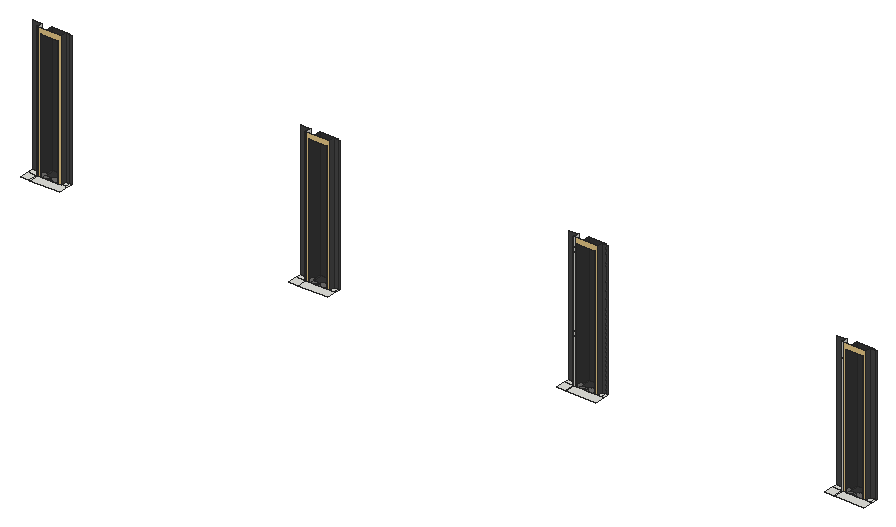
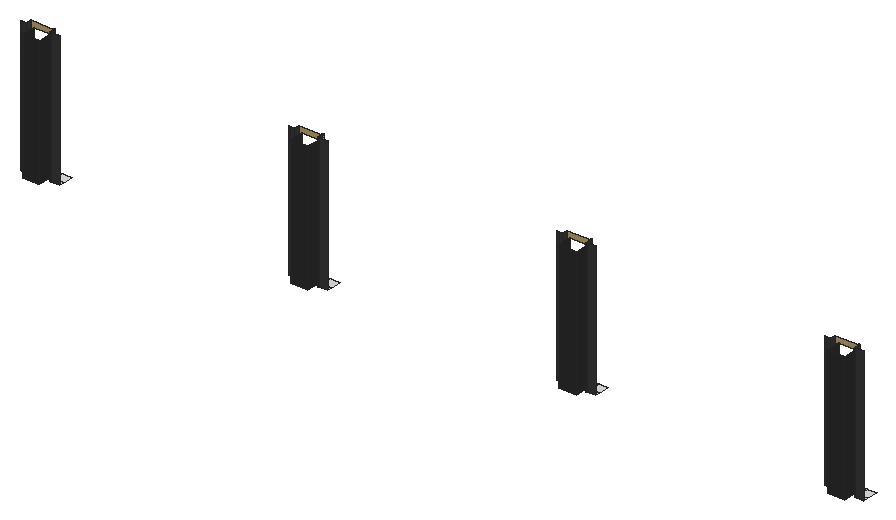
# SketchUp Ruby script. Lengths in inches.
U = 1.inch
M = Sketchup.active_model
def pt(a) = Geom::Point3d.new(a.map { |v| v * U })
def face(e, loops, mat)
  f = e.add_face(loops[0].map { |a| pt(a) })
  loops[1..].each { |l| e.add_face(l.map { |a| pt(a) }).erase! }
  f.material = f.back_material = mat if mat
  f
end
# faces: each face lists its corners as indices into pts; further lists are holes
def faces(e, pts, list, mat = nil) = list.each { |f| face(e, (f[0].is_a?(Array) ? f : [f]).map { |l| l.map { |i| pts[i] } }, mat) }
# xy, xz, yz: faces in a plane at the given z, y or x. An outline is a flat list of corners, or four numbers for a rectangle; further outlines are holes
def ring(l) = l.size == 4 ? [[l[0], l[1]], [l[2], l[1]], [l[2], l[3]], [l[0], l[3]]] : l.each_slice(2).to_a
def flat(e, list, mat, &to3) = list.each { |f| face(e, (f[0].is_a?(Array) ? f : [f]).map { |l| ring(l).map { |u, v| to3.(u, v) } }, mat) }
def xy(e, z, list, mat = nil) = flat(e, list, mat) { |x, y| [x, y, z] }
def xz(e, y, list, mat = nil) = flat(e, list, mat) { |x, z| [x, y, z] }
def yz(e, x, list, mat = nil) = flat(e, list, mat) { |y, z| [x, y, z] }
def lines(e, pts, list) = list.each { |a, b| e.add_line(pt(pts[a]), pt(pts[b])) }
# prism: a flat outline (further loops are holes) pulled along v
def prism(e, loops, v, mat = nil)
  f = face(e, loops, mat); d = Geom::Vector3d.new(v.map { |x| x * U })
  f.pushpull(f.normal.samedirection?(d) ? d.length : -d.length)
end
def box(e, o, s, mat = nil) = prism(e, [[o, [o[0] + s[0], o[1], o[2]], [o[0] + s[0], o[1] + s[1], o[2]], [o[0], o[1] + s[1], o[2]]]], [0, 0, s[2]], mat)
def at(x, y, z, deg = 0) = Geom::Transformation.translation(pt([x, y, z])) * Geom::Transformation.rotation(ORIGIN, Z_AXIS, deg.degrees)
def axes(o, x, y, z) = Geom::Transformation.new([*x, 0, *y, 0, *z, 0, *pt(o).to_a, 1])
def part(name) = M.definitions.add(name)
# library, detail: a bought-in or finely detailed component or shape, given as its bounding box
def library(name, o, s) = part(name).tap { |d| box(d.entities, o, s) }
def detail(e, o, s) = box(e.add_group.entities, o, s)
def put(e, d, t, mat = nil) = e.add_instance(d, t).tap { |i| i.material = mat if mat }
def group(e, t, mat = nil) = e.add_group.tap { |g| g.transformation = t; g.material = mat if mat }.entities
root = M.entities
M.materials.add("[0043_SaddleBrown]4").color = [124, 123, 122]
M.materials.add("[Granite Dark Gray]").color = [69, 68, 68]
M.materials.add("[Slate Light Tile]").color = [54, 54, 54]
M.materials.add("[Stone Brushed Khaki]").color = [226, 197, 133]
xy(root,161.375,[[310,542.125,351.59,589.17],[351.59,542.125,354.34,585.86],[354.34,542.125,492.21,589.17],[1560.62,542.125,1602.22,589.17],[1602.22,542.125,1604.97,585.86],
  [1604.97,542.125,1742.84,589.17],[2811.25,542.125,2852.84,589.17],[2852.84,542.125,2855.59,585.86],[2855.59,542.125,2993.46,589.17],[4061.87,542.125,4103.47,589.17],
  [4103.47,542.125,4106.22,585.86],[4106.22,542.125,4244.09,589.17],[351.59,585.86,354.34,589.17],[1602.22,585.86,1604.97,589.17],[2852.84,585.86,2855.59,589.17],
  [4103.47,585.86,4106.22,589.17],[310,589.17,351.59,613.74],[351.59,589.17,354.34,613.74],[464.1,589.17,482.97,613.74],[482.97,589.17,492.21,613.74],
  [1560.62,589.17,1602.22,613.74],[1602.22,589.17,1604.97,613.74],[1714.72,589.17,1733.59,613.74],[1733.59,589.17,1742.84,613.74],[2811.25,589.17,2852.84,613.74],
  [2852.84,589.17,2855.59,613.74],[2965.35,589.17,2984.22,613.74],[2984.22,589.17,2993.46,613.74],[4061.87,589.17,4103.47,613.74],[4103.47,589.17,4106.22,613.74],
  [4215.97,589.17,4234.84,613.74],[4234.84,589.17,4244.09,613.74]])
xy(root,161.375,[[367.98,589.17,376.61,653.8],[376.61,589.17,449.07,653.8],[1618.6,589.17,1627.23,653.8],[1627.23,589.17,1699.7,653.8],[2869.23,589.17,2877.86,653.8],
  [2877.86,589.17,2950.32,653.8],[4119.85,589.17,4128.48,653.8],[4128.48,589.17,4200.95,653.8]],"[Slate Light Tile]")
xz(root,585.86,[[351.59,161.375,354.34,785.86],[1602.22,161.375,1604.97,785.86],[2852.84,161.375,2855.59,785.86],[4103.47,161.375,4106.22,785.86]],"[Granite Dark Gray]")
xz(root,589.17,[[351.59,161.375,354.34,784.4375],[1602.22,161.375,1604.97,784.4375],[2852.84,161.375,2855.59,784.4375],[4103.47,161.375,4106.22,784.4375]])
xz(root,589.17,[[367.98,161.375,367.98,162.26,369.0625,163.14,369.98,164.125,370.71,165.18,371.24,166.31,371.5625,167.47,371.67,168.65,371.5625,169.83,371.24,170.99,370.71,172.11,369.98,173.17,369.0625,174.15,367.98,175.04,367.98,176.23,369.45,176.45,370.9,176.73,372.33,177.07,373.74,177.46,375.11,177.91,376.44,178.41,377.73,178.96,378.98,179.57,380.1875,180.22,381.34,180.92,382.43,181.66,383.47,182.45,384.12,182.92,384.84,183.34,385.61,183.7,386.4375,184,387.3,184.23,388.19,184.4,389.11,184.5,390.03,184.53,390.95,184.49,391.86,184.375,392.75,184.19,393.6,183.95,393.91,183.83,394.2,183.7,394.47,183.56,394.73,183.39,394.96,183.21,395.18,183.02,395.37,182.82,395.54,182.6,395.68,182.375,395.79,182.14,395.88,181.9,395.94,181.66,395.97,181.42,395.95,181.18,395.9,180.94,395.82,180.71,395.69,180.49,395.54,180.28,395.34,180.08,395.125,179.9,394.875,179.74,394.6,179.6,394.3125,179.48,394,179.39,393.8125,179.64,393.61,179.88,393.39,180.12,393.16,180.35,392.93,180.57,392.68,180.79,392.42,181.01,392.15,181.21,391.87,181.41,391.58,181.6,391.28,181.79,390.97,181.96,390.55,181.9,390.14,181.8,389.74,181.67,389.36,181.52,389,181.34,388.67,181.14,388.36,180.92,388.09,180.67,387.86,180.41,387.66,180.13,387.49,179.84,387.37,179.54,387.23,179.07,387.12,178.59,387.04,178.11,387,177.63,386.99,177.15,387.01,176.66,387.0625,176.18,387.15,175.7,387.27,175.23,387.42,174.76,387.6,174.29,387.82,173.83,386.35,173.43,384.9375,172.94,383.59,172.35,382.32,171.68,381.14,170.93,380.06,170.11,379.08,169.23,378.21,168.28,377.47,167.28,376.85,166.24,376.36,165.16,376.01,164.06,375.63,163.88,374.89,163.5,374.54,163.3,374.1875,163.09,373.85,162.87,373.52,162.64,373.2,162.41,372.89,162.17,372.59,161.93,372.3,161.67,372.02,161.375],[380.49,161.375,381.93,164.8,384.38,167.82,387.74,170.36,391.8125,172.26,396.38,173.45,401.21,173.84,406.03,173.43,410.59,172.22,414.65,170.3,417.98,167.75,420.41,164.72,421.8125,161.375,415.66,161.375,414.48,163.56,412.67,165.52,410.32,167.15,407.53,168.37,404.45,169.14,401.2,169.4,397.96,169.16,394.86,168.41,392.0625,167.2,389.69,165.59,387.86,163.64,386.65,161.375],[393.03,161.375,393.92,162.48,395.09,163.4375,396.48,164.22,398.0625,164.8,399.76,165.16,401.52,165.28,403.29,165.16,404.99,164.8,406.5625,164.22,407.96,163.4375,409.125,162.48,410.02,161.375],[1618.6,161.375,1618.6,162.26,1619.6875,163.14,1620.6,164.125,1621.33,165.18,1621.86,166.31,1622.1875,167.47,1622.29,168.65,1622.1875,169.83,1621.86,170.99,1621.33,172.11,1620.6,173.17,1619.6875,174.15,1618.6,175.04,1618.6,176.23,1620.07,176.45,1621.53,176.73,1622.96,177.07,1624.36,177.46,1625.73,177.91,1627.07,178.41,1628.36,178.96,1629.61,179.57,1630.8125,180.22,1631.96,180.92,1633.06,181.66,1634.09,182.45,1634.75,182.92,1635.46,183.34,1636.24,183.7,1637.0625,184,1637.93,184.23,1638.82,184.4,1639.73,184.5,1640.65,184.53,1641.57,184.49,1642.48,184.375,1643.37,184.19,1644.23,183.95,1644.53,183.83,1644.82,183.7,1645.1,183.56,1645.35,183.39,1645.59,183.21,1645.8,183.02,1645.99,182.82,1646.16,182.6,1646.3,182.375,1646.42,182.14,1646.51,181.9,1646.57,181.66,1646.59,181.42,1646.58,181.18,1646.53,180.94,1646.44,180.71,1646.32,180.49,1646.16,180.28,1645.97,180.08,1645.75,179.9,1645.5,179.74,1645.23,179.6,1644.9375,179.48,1644.63,179.39,1644.4375,179.64,1644.23,179.88,1644.02,180.12,1643.79,180.35,1643.55,180.57,1643.3,180.79,1643.04,181.01,1642.77,181.21,1642.49,181.41,1641.91,181.79,1641.6,181.96,1641.17,181.9,1640.76,181.8,1640.36,181.67,1639.98,181.52,1639.625,181.34,1639.29,181.14,1638.99,180.92,1638.72,180.67,1638.48,180.41,1638.28,180.13,1638.12,179.84,1637.99,179.54,1637.85,179.07,1637.74,178.59,1637.67,178.11,1637.62,177.63,1637.61,177.15,1637.63,176.66,1637.6875,176.18,1637.77,175.7,1637.89,175.23,1638.04,174.76,1638.23,174.29,1638.44,173.83,1636.97,173.43,1635.5625,172.94,1634.21,172.35,1632.95,171.68,1631.76,170.93,1630.68,170.11,1629.7,169.23,1628.84,168.28,1628.09,167.28,1627.47,166.24,1626.99,165.16,1626.63,164.06,1626.25,163.88,1625.88,163.69,1625.52,163.5,1625.16,163.3,1624.8125,163.09,1624.47,162.87,1624.14,162.64,1623.82,162.41,1623.51,162.17,1623.22,161.93,1622.93,161.67,1622.65,161.375],[1631.12,161.375,1632.55,164.8,1635.01,167.82,1638.36,170.36,1642.4375,172.26,1647.01,173.45,1651.83,173.84,1656.66,173.43,1661.22,172.22,1665.27,170.3,1668.6,167.75,1671.04,164.72,1672.4375,161.375,1666.28,161.375,1665.1,163.56,1663.29,165.52,1660.94,167.15,1658.16,168.37,1655.07,169.14,1651.83,169.4,1648.58,169.16,1645.49,168.41,1642.6875,167.2,1640.32,165.59,1638.48,163.64,1637.28,161.375],
  [1643.65,161.375,1644.55,162.48,1645.71,163.4375,1647.11,164.22,1648.6875,164.8,1650.39,165.16,1652.15,165.28,1653.91,165.16,1655.61,164.8,1657.1875,164.22,1658.58,163.4375,1659.75,162.48,1660.65,161.375],[2869.23,161.375,2869.23,162.26,2870.3125,163.14,2871.23,164.125,2871.96,165.18,2872.49,166.31,2872.8125,167.47,2872.92,168.65,2872.8125,169.83,2872.49,170.99,2871.96,172.11,2871.23,173.17,2870.3125,174.15,2869.23,175.04,2869.23,176.23,2870.7,176.45,2872.15,176.73,2873.58,177.07,2874.99,177.46,2876.36,177.91,2877.69,178.41,2878.98,178.96,2880.23,179.57,2881.4375,180.22,2882.59,180.92,2883.68,181.66,2884.72,182.45,2885.37,182.92,2886.09,183.34,2886.86,183.7,2887.6875,184,2888.55,184.23,2889.44,184.4,2890.36,184.5,2891.28,184.53,2892.2,184.49,2893.11,184.375,2894,184.19,2894.85,183.95,2895.16,183.83,2895.45,183.7,2895.72,183.56,2895.98,183.39,2896.21,183.21,2896.43,183.02,2896.62,182.82,2896.79,182.6,2896.93,182.375,2897.04,182.14,2897.13,181.9,2897.19,181.66,2897.22,181.42,2897.2,181.18,2897.15,180.94,2897.07,180.71,2896.94,180.49,2896.79,180.28,2896.59,180.08,2896.375,179.9,2896.125,179.74,2895.85,179.6,2895.5625,179.48,2895.25,179.39,2895.0625,179.64,2894.86,179.88,2894.64,180.12,2894.41,180.35,2894.18,180.57,2893.93,180.79,2893.67,181.01,2893.4,181.21,2893.12,181.41,2892.83,181.6,2892.53,181.79,2892.22,181.96,2891.8,181.9,2891.39,181.8,2890.99,181.67,2890.61,181.52,2890.25,181.34,2889.92,181.14,2889.61,180.92,2889.34,180.67,2889.11,180.41,2888.91,180.13,2888.74,179.84,2888.62,179.54,2888.48,179.07,2888.37,178.59,2888.29,178.11,2888.25,177.63,2888.24,177.15,2888.26,176.66,2888.3125,176.18,2888.4,175.7,2888.52,175.23,2888.67,174.76,2888.85,174.29,2889.07,173.83,2887.6,173.43,2886.1875,172.94,2884.84,172.35,2883.57,171.68,2882.39,170.93,2881.31,170.11,2880.33,169.23,2879.46,168.28,2878.72,167.28,2878.1,166.24,2877.61,165.16,2877.26,164.06,2876.88,163.88,2876.14,163.5,2875.79,163.3,2875.4375,163.09,2875.1,162.87,2874.77,162.64,2874.45,162.41,2874.14,162.17,2873.84,161.93,2873.55,161.67,2873.27,161.375],[2881.74,161.375,2883.18,164.8,2885.63,167.82,2888.99,170.36,2893.0625,172.26,2897.63,173.45,2902.46,173.84,2907.28,173.43,2911.84,172.22,2915.9,170.3,2919.23,167.75,2921.66,164.72,2923.0625,161.375,2916.91,161.375,2915.73,163.56,2913.92,165.52,2911.57,167.15,2908.78,168.37,2905.7,169.14,2902.45,169.4,2899.21,169.16,2896.11,168.41,2893.3125,167.2,2890.94,165.59,2889.11,163.64,2887.9,161.375],[2894.28,161.375,2895.17,162.48,2896.34,163.4375,2897.73,164.22,2899.3125,164.8,2901.01,165.16,2902.77,165.28,2904.54,165.16,2906.24,164.8,2907.8125,164.22,2909.21,163.4375,2910.375,162.48,2911.27,161.375],[4119.85,161.375,4119.85,162.26,4120.9375,163.14,4121.85,164.125,4122.58,165.18,4123.11,166.31,4123.4375,167.47,4123.54,168.65,4123.4375,169.83,4123.11,170.99,4122.58,172.11,4121.85,173.17,4120.9375,174.15,4119.85,175.04,4119.85,176.23,4121.32,176.45,4122.78,176.73,4124.21,177.07,4125.61,177.46,4126.98,177.91,4128.32,178.41,4129.61,178.96,4130.86,179.57,4132.0625,180.22,4133.21,180.92,4134.31,181.66,4135.34,182.45,4136,182.92,4136.71,183.34,4137.49,183.7,4138.3125,184,4139.18,184.23,4140.07,184.4,4140.98,184.5,4141.9,184.53,4142.82,184.49,4143.73,184.375,4144.62,184.19,4145.48,183.95,4145.78,183.83,4146.07,183.7,4146.35,183.56,4146.6,183.39,4146.84,183.21,4147.05,183.02,4147.24,182.82,4147.41,182.6,4147.55,182.375,4147.67,182.14,4147.76,181.9,4147.82,181.66,4147.84,181.42,4147.83,181.18,4147.78,180.94,4147.69,180.71,4147.57,180.49,4147.41,180.28,4147.22,180.08,4147,179.9,4146.75,179.74,4146.48,179.6,4146.1875,179.48,4145.88,179.39,4145.6875,179.64,4145.48,179.88,4145.27,180.12,4145.04,180.35,4144.8,180.57,4144.55,180.79,4144.29,181.01,4144.02,181.21,4143.74,181.41,4143.16,181.79,4142.85,181.96,4142.42,181.9,4142.01,181.8,4141.61,181.67,4141.23,181.52,4140.875,181.34,4140.54,181.14,4140.24,180.92,4139.97,180.67,4139.73,180.41,4139.53,180.13,4139.37,179.84,4139.24,179.54,4139.1,179.07,4138.99,178.59,4138.92,178.11,4138.87,177.63,4138.86,177.15,4138.88,176.66,4138.9375,176.18,4139.02,175.7,4139.14,175.23,4139.29,174.76,4139.48,174.29,4139.69,173.83,4138.22,173.43,4136.8125,172.94,4135.46,172.35,4134.2,171.68,4133.01,170.93,4131.93,170.11,4130.95,169.23,4130.09,168.28,4129.34,167.28,4128.72,166.24,4128.24,165.16,4127.88,164.06,4127.5,163.88,4127.13,163.69,4126.77,163.5,4126.41,163.3,4126.0625,163.09,4125.72,162.87,4125.39,162.64,4125.07,162.41,4124.76,162.17,4124.47,161.93,4124.18,161.67,4123.9,161.375],
  [4132.37,161.375,4133.8,164.8,4136.26,167.82,4139.61,170.36,4143.6875,172.26,4148.26,173.45,4153.08,173.84,4157.91,173.43,4162.47,172.22,4166.52,170.3,4169.85,167.75,4172.29,164.72,4173.6875,161.375,4167.53,161.375,4166.35,163.56,4164.54,165.52,4162.19,167.15,4159.41,168.37,4156.32,169.14,4153.08,169.4,4149.83,169.16,4146.74,168.41,4143.9375,167.2,4141.57,165.59,4139.73,163.64,4138.53,161.375],[4144.9,161.375,4145.8,162.48,4146.96,163.4375,4148.36,164.22,4149.9375,164.8,4151.64,165.16,4153.4,165.28,4155.16,165.16,4156.86,164.8,4158.4375,164.22,4159.83,163.4375,4161,162.48,4161.9,161.375],[432.01,162.27,430.35,162.39,428.74,162.68,427.2,163.15,425.77,163.78,424.49,164.55,423.38,165.45,422.47,166.46,421.78,167.55,421.32,168.71,421.1,169.9,421.13,171.1,421.08,171.86,421.16,172.62,421.37,173.37,421.7,174.09,422.15,174.78,422.72,175.42,423.39,176.01,424.15,176.54,425,176.99,425.91,177.37,426.89,177.66,427.9,177.87,428.58,178.16,429.31,178.36,430.09,178.47,430.875,178.48,431.65,178.4,432.4,178.22,433.09,177.95,433.71,177.6,434.24,177.19,434.67,176.71,434.97,176.18,435.15,175.63,435.55,175.22,435.84,174.77,436.03,174.29,436.09,173.8,436.04,173.3,435.87,172.82,435.58,172.36,435.2,171.95,434.72,171.59,434.16,171.3,433.53,171.08,432.87,170.9375,432.64,171.19,432.39,171.43,432.14,171.66,431.875,171.89,431.6,172.11,431.3125,172.33,431.02,172.53,430.4,172.93,429.74,173.29,429.4,173.46,429.03,173.29,428.69,173.09,428.37,172.87,428.09,172.625,427.85,172.36,427.66,172.07,427.5,171.78,427.39,171.47,427.33,171.15,427.32,170.84,427.35,170.52,427.43,170.21,427.72,169.58,428.14,168.99,428.6875,168.47,429.35,168.01,430.1,167.63,430.93,167.35,431.81,167.16,432.72,167.08,433.63,167.11,434.53,167.25,435.39,167.48,436.18,167.8125,437.6,168.63,438.85,169.58,439.91,170.64,440.76,171.79,441.39,173.02,441.78,174.29,441.93,175.59,441.84,176.9,441.5,178.18,440.93,179.42,440.12,180.6,439.11,181.68,439.89,181.55,440.68,181.45,441.48,181.4,442.28,181.38,443.08,181.41,443.88,181.47,444.67,181.57,445.45,181.72,446.21,181.9,446.95,182.12,447.67,182.375,448.37,182.67,448.37,173.66,447.95,172.32,447.36,171.03,446.6,169.77,445.67,168.58,444.59,167.46,443.36,166.42,442,165.46,440.52,164.61,438.94,163.86,437.26,163.23,435.5,162.72,433.68,162.33],[1682.64,162.27,1680.98,162.39,1679.36,162.68,1677.82,163.15,1676.4,163.78,1675.11,164.55,1674.01,165.45,1673.09,166.46,1672.4,167.55,1671.94,168.71,1671.72,169.9,1671.75,171.1,1671.7,171.86,1671.79,172.62,1671.99,173.37,1672.33,174.09,1672.78,174.78,1673.34,175.42,1674.01,176.01,1674.78,176.54,1675.62,176.99,1676.54,177.37,1677.51,177.66,1678.53,177.87,1679.2,178.16,1679.94,178.36,1680.71,178.47,1681.5,178.48,1682.28,178.4,1683.02,178.22,1683.72,177.95,1684.34,177.6,1684.87,177.19,1685.29,176.71,1685.6,176.18,1685.77,175.63,1686.17,175.22,1686.47,174.77,1686.65,174.29,1686.72,173.8,1686.66,173.3,1686.49,172.82,1686.21,172.36,1685.82,171.95,1685.34,171.59,1684.78,171.3,1684.16,171.08,1683.5,170.9375,1683.26,171.19,1683.02,171.43,1682.5,171.89,1682.22,172.11,1681.9375,172.33,1681.64,172.53,1681.34,172.73,1681.02,172.93,1680.7,173.11,1680.37,173.29,1680.03,173.46,1679.66,173.29,1679.31,173.09,1679,172.87,1678.72,172.625,1678.48,172.36,1678.28,172.07,1678.13,171.78,1678.02,171.47,1677.96,171.15,1677.94,170.84,1677.97,170.52,1678.06,170.21,1678.34,169.58,1678.77,168.99,1679.3125,168.47,1679.97,168.01,1680.73,167.63,1681.55,167.35,1682.43,167.16,1683.34,167.08,1684.26,167.11,1685.16,167.25,1686.01,167.48,1686.8,167.8125,1688.22,168.63,1689.47,169.58,1690.53,170.64,1691.39,171.79,1692.01,173.02,1692.41,174.29,1692.56,175.59,1692.46,176.9,1692.125,178.18,1691.55,179.42,1690.75,180.6,1689.73,181.68,1690.51,181.55,1691.3,181.45,1692.1,181.4,1692.91,181.38,1693.71,181.41,1694.51,181.47,1695.3,181.57,1696.07,181.72,1696.83,181.9,1697.58,182.12,1698.3,182.375,1698.99,182.67,1698.99,173.66,1698.58,172.32,1697.98,171.03,1697.22,169.77,1696.3,168.58,1695.21,167.46,1693.99,166.42,1692.63,165.46,1691.15,164.61,1689.56,163.86,1687.88,163.23,1686.125,162.72,1684.31,162.33],[2933.26,162.27,2931.6,162.39,2929.99,162.68,2928.45,163.15,2927.02,163.78,2925.74,164.55,2924.63,165.45,2923.72,166.46,2923.03,167.55,2922.57,168.71,2922.35,169.9,2922.38,171.1,2922.33,171.86,2922.41,172.62,2922.62,173.37,2922.95,174.09,2923.4,174.78,2923.97,175.42,2924.64,176.01,2925.4,176.54,2926.25,176.99,2927.16,177.37,2928.14,177.66,2929.15,177.87,2929.83,178.16,2930.56,178.36,2931.34,178.47,2932.125,178.48,2932.9,178.4,2933.65,178.22,2934.34,177.95,2934.96,177.6,2935.49,177.19,2935.92,176.71,2936.22,176.18,2936.4,175.63,2936.8,175.22,2937.09,174.77,2937.28,174.29,2937.34,173.8,2937.29,173.3,2937.12,172.82,2936.83,172.36,2936.45,171.95,2935.97,171.59,2935.41,171.3,2934.78,171.08,2934.12,170.9375,2933.89,171.19,2933.64,171.43,2933.39,171.66,2933.125,171.89,2932.85,172.11,2932.5625,172.33,2932.27,172.53,2931.65,172.93,2930.99,173.29,2930.65,173.46,2930.28,173.29,2929.94,173.09,2929.62,172.87,2929.34,172.625,2929.1,172.36,2928.91,172.07,2928.75,171.78,2928.64,171.47,2928.58,171.15,2928.57,170.84,2928.6,170.52,2928.68,170.21,2928.97,169.58,2929.39,168.99,2929.9375,168.47,2930.6,168.01,2931.35,167.63,2932.18,167.35,2933.06,167.16,2933.97,167.08,2934.88,167.11,2935.78,167.25,2936.64,167.48,2937.43,167.8125,2938.85,168.63,2940.1,169.58,2941.16,170.64,2942.01,171.79,2942.64,173.02,2943.03,174.29,2943.18,175.59,2943.09,176.9,2942.75,178.18,2942.18,179.42,2941.37,180.6,2940.36,181.68,2941.14,181.55,2941.93,181.45,2942.73,181.4,2943.53,181.38,2944.33,181.41,2945.13,181.47,2945.92,181.57,2946.7,181.72,2947.46,181.9,2948.2,182.12,2948.92,182.375,2949.62,182.67,2949.62,173.66,2949.2,172.32,2948.61,171.03,2947.85,169.77,2946.92,168.58,2945.84,167.46,2944.61,166.42,2943.25,165.46,2941.77,164.61,2940.19,163.86,2938.51,163.23,2936.75,162.72,2934.93,162.33],
  [4183.89,162.27,4182.23,162.39,4180.61,162.68,4179.07,163.15,4177.65,163.78,4176.36,164.55,4175.26,165.45,4174.34,166.46,4173.65,167.55,4173.19,168.71,4172.97,169.9,4173,171.1,4172.95,171.86,4173.04,172.62,4173.24,173.37,4173.58,174.09,4174.03,174.78,4174.59,175.42,4175.26,176.01,4176.03,176.54,4176.87,176.99,4177.79,177.37,4178.76,177.66,4179.78,177.87,4180.45,178.16,4181.19,178.36,4181.96,178.47,4182.75,178.48,4183.53,178.4,4184.27,178.22,4184.97,177.95,4185.59,177.6,4186.12,177.19,4186.54,176.71,4186.85,176.18,4187.02,175.63,4187.42,175.22,4187.72,174.77,4187.9,174.29,4187.97,173.8,4187.91,173.3,4187.74,172.82,4187.46,172.36,4187.07,171.95,4186.59,171.59,4186.03,171.3,4185.41,171.08,4184.75,170.9375,4184.51,171.19,4184.27,171.43,4183.75,171.89,4183.47,172.11,4183.1875,172.33,4182.89,172.53,4182.59,172.73,4182.27,172.93,4181.95,173.11,4181.62,173.29,4181.28,173.46,4180.91,173.29,4180.56,173.09,4180.25,172.87,4179.97,172.625,4179.73,172.36,4179.53,172.07,4179.38,171.78,4179.27,171.47,4179.21,171.15,4179.19,170.84,4179.22,170.52,4179.31,170.21,4179.59,169.58,4180.02,168.99,4180.5625,168.47,4181.22,168.01,4181.98,167.63,4182.8,167.35,4183.68,167.16,4184.59,167.08,4185.51,167.11,4186.41,167.25,4187.26,167.48,4188.05,167.8125,4189.47,168.63,4190.72,169.58,4191.78,170.64,4192.64,171.79,4193.26,173.02,4193.66,174.29,4193.81,175.59,4193.71,176.9,4193.375,178.18,4192.8,179.42,4192,180.6,4190.98,181.68,4191.76,181.55,4192.55,181.45,4193.35,181.4,4194.16,181.38,4194.96,181.41,4195.76,181.47,4196.55,181.57,4197.32,181.72,4198.08,181.9,4198.83,182.12,4199.55,182.375,4200.24,182.67,4200.24,173.66,4199.83,172.32,4199.23,171.03,4198.47,169.77,4197.55,168.58,4196.46,167.46,4195.24,166.42,4193.88,165.46,4192.4,164.61,4190.81,163.86,4189.13,163.23,4187.375,162.72,4185.56,162.33]],"[0043_SaddleBrown]4")
xz(root,589.17,[[354.34,161.375,367.98,161.375,367.98,759.44,449.07,759.44,449.07,161.375,464.1,161.375,464.1,784.4375,354.34,784.4375],[1604.97,161.375,1618.6,161.375,1618.6,759.44,1699.7,759.44,1699.7,161.375,1714.72,161.375,1714.72,784.4375,1604.97,784.4375],[2855.59,161.375,2869.23,161.375,2869.23,759.44,2950.32,759.44,2950.32,161.375,2965.35,161.375,2965.35,784.4375,2855.59,784.4375],[4106.22,161.375,4119.85,161.375,4119.85,759.44,4200.95,759.44,4200.95,161.375,4215.97,161.375,4215.97,784.4375,4106.22,784.4375]],"[Stone Brushed Khaki]")
xz(root,613.74,[[351.59,161.375,354.34,784.4375],[1602.22,161.375,1604.97,784.4375],[2852.84,161.375,2855.59,784.4375],[4103.47,161.375,4106.22,784.4375]])
xz(root,613.74,[[310,161.375,351.59,784.4375],[464.1,161.375,482.97,784.4375],[482.97,161.375,492.21,784.4375],[1560.62,161.375,1602.22,784.4375],[1714.72,161.375,1733.59,784.4375],
  [1733.59,161.375,1742.84,784.4375],[2811.25,161.375,2852.84,784.4375],[2965.35,161.375,2984.22,784.4375],[2984.22,161.375,2993.46,784.4375],[4061.87,161.375,4103.47,784.4375],
  [4215.97,161.375,4234.84,784.4375],[4234.84,161.375,4244.09,784.4375]],"[Granite Dark Gray]")
xz(root,653.8,[[367.98,161.375,449.07,759.44],[1618.6,161.375,1699.7,759.44],[2869.23,161.375,2950.32,759.44],[4119.85,161.375,4200.95,759.44]],"[Slate Light Tile]")
yz(root,351.59,[[585.86,161.375,589.17,785.86]])
yz(root,351.59,[[589.17,161.375,613.74,784.4375]],"[Granite Dark Gray]")
yz(root,354.34,[[585.86,161.375,589.17,785.86],[589.17,161.375,613.74,784.4375]])
yz(root,367.98,[[589.17,161.375,653.8,759.44]],"[Slate Light Tile]")
yz(root,449.07,[[589.17,161.375,653.8,759.44]],"[Slate Light Tile]")
yz(root,464.1,[[589.17,161.375,613.74,784.4375]],"[Granite Dark Gray]")
yz(root,1602.22,[[585.86,161.375,589.17,785.86]])
yz(root,1602.22,[[589.17,161.375,613.74,784.4375]],"[Granite Dark Gray]")
yz(root,1604.97,[[585.86,161.375,589.17,785.86],[589.17,161.375,613.74,784.4375]])
yz(root,1618.6,[[589.17,161.375,653.8,759.44]],"[Slate Light Tile]")
yz(root,1699.7,[[589.17,161.375,653.8,759.44]],"[Slate Light Tile]")
yz(root,1714.72,[[589.17,161.375,613.74,784.4375]],"[Granite Dark Gray]")
yz(root,2852.84,[[585.86,161.375,589.17,785.86]])
yz(root,2852.84,[[589.17,161.375,613.74,784.4375]],"[Granite Dark Gray]")
yz(root,2855.59,[[585.86,161.375,589.17,785.86],[589.17,161.375,613.74,784.4375]])
yz(root,2869.23,[[589.17,161.375,653.8,759.44]],"[Slate Light Tile]")
yz(root,2950.32,[[589.17,161.375,653.8,759.44]],"[Slate Light Tile]")
yz(root,2965.35,[[589.17,161.375,613.74,784.4375]],"[Granite Dark Gray]")
yz(root,4103.47,[[585.86,161.375,589.17,785.86]])
yz(root,4103.47,[[589.17,161.375,613.74,784.4375]],"[Granite Dark Gray]")
yz(root,4106.22,[[585.86,161.375,589.17,785.86],[589.17,161.375,613.74,784.4375]])
yz(root,4119.85,[[589.17,161.375,653.8,759.44]],"[Slate Light Tile]")
yz(root,4200.95,[[589.17,161.375,653.8,759.44]],"[Slate Light Tile]")
yz(root,4215.97,[[589.17,161.375,613.74,784.4375]],"[Granite Dark Gray]")
